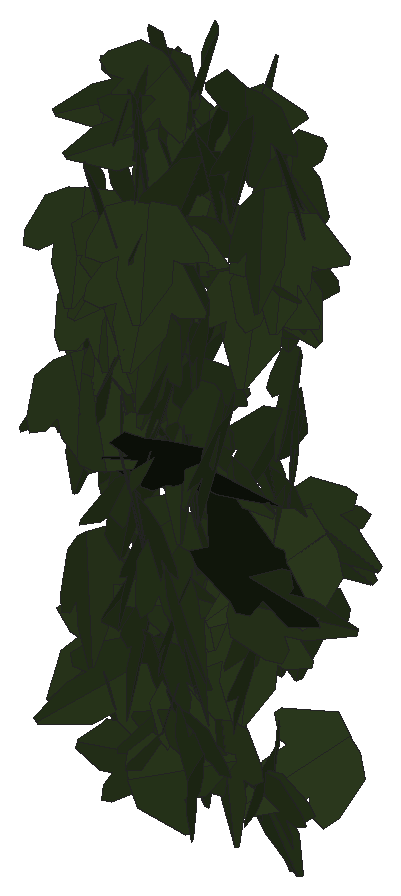
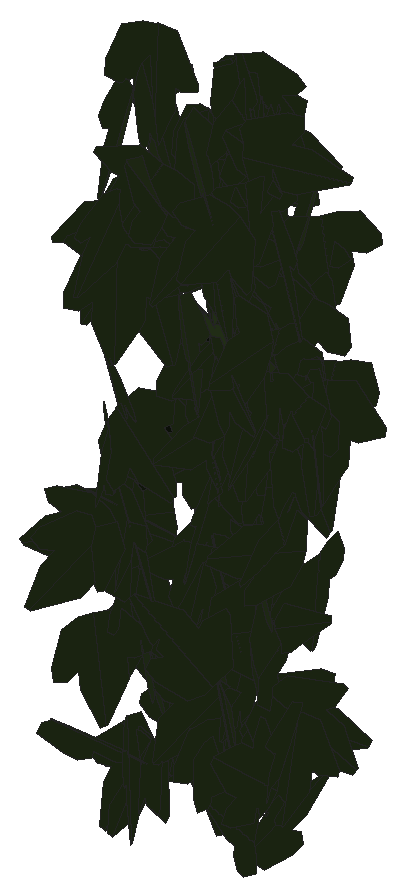
# SketchUp Ruby script. Lengths in inches.
U = 1.inch
M = Sketchup.active_model
def pt(a) = Geom::Point3d.new(a.map { |v| v * U })
def face(e, loops, mat)
  f = e.add_face(loops[0].map { |a| pt(a) })
  loops[1..].each { |l| e.add_face(l.map { |a| pt(a) }).erase! }
  f.material = f.back_material = mat if mat
  f
end
# faces: each face lists its corners as indices into pts; further lists are holes
def faces(e, pts, list, mat = nil) = list.each { |f| face(e, (f[0].is_a?(Array) ? f : [f]).map { |l| l.map { |i| pts[i] } }, mat) }
# xy, xz, yz: faces in a plane at the given z, y or x. An outline is a flat list of corners, or four numbers for a rectangle; further outlines are holes
def ring(l) = l.size == 4 ? [[l[0], l[1]], [l[2], l[1]], [l[2], l[3]], [l[0], l[3]]] : l.each_slice(2).to_a
def flat(e, list, mat, &to3) = list.each { |f| face(e, (f[0].is_a?(Array) ? f : [f]).map { |l| ring(l).map { |u, v| to3.(u, v) } }, mat) }
def xy(e, z, list, mat = nil) = flat(e, list, mat) { |x, y| [x, y, z] }
def xz(e, y, list, mat = nil) = flat(e, list, mat) { |x, z| [x, y, z] }
def yz(e, x, list, mat = nil) = flat(e, list, mat) { |y, z| [x, y, z] }
def lines(e, pts, list) = list.each { |a, b| e.add_line(pt(pts[a]), pt(pts[b])) }
# prism: a flat outline (further loops are holes) pulled along v
def prism(e, loops, v, mat = nil)
  f = face(e, loops, mat); d = Geom::Vector3d.new(v.map { |x| x * U })
  f.pushpull(f.normal.samedirection?(d) ? d.length : -d.length)
end
def box(e, o, s, mat = nil) = prism(e, [[o, [o[0] + s[0], o[1], o[2]], [o[0] + s[0], o[1] + s[1], o[2]], [o[0], o[1] + s[1], o[2]]]], [0, 0, s[2]], mat)
def at(x, y, z, deg = 0) = Geom::Transformation.translation(pt([x, y, z])) * Geom::Transformation.rotation(ORIGIN, Z_AXIS, deg.degrees)
def axes(o, x, y, z) = Geom::Transformation.new([*x, 0, *y, 0, *z, 0, *pt(o).to_a, 1])
def part(name) = M.definitions.add(name)
# library, detail: a bought-in or finely detailed component or shape, given as its bounding box
def library(name, o, s) = part(name).tap { |d| box(d.entities, o, s) }
def detail(e, o, s) = box(e.add_group.entities, o, s)
def put(e, d, t, mat = nil) = e.add_instance(d, t).tap { |i| i.material = mat if mat }
def group(e, t, mat = nil) = e.add_group.tap { |g| g.transformation = t; g.material = mat if mat }.entities
root = M.entities
M.materials.add("efeu1").color = [18, 25, 13]
M.materials.add("efeu2").color = [43, 57, 29]
c1 = part("ivyleaf_10")
p = [[0,0.5,-0.03],[-0.0625,2.02,-0.43],[-0.19,2.01,-0.46],[-0.54,1.05,-0.29],[-0.52,0.625,-0.18],[-0.83,0.76,-0.28],
  [-1.16,0.64,-0.33],[-1.15,0.33,-0.24],[-0.77,-0.39,0.02],[-0.3,-0.51,0.16],[0.04,-0.48,0.23],[-0.02,2.01,-0.4375],
  [-0.06,2.01,-0.43],[0.04,-0.49,0.23],[0.67,-0.49,0.14],[1.38,0.36,-0.2],[1.375,0.51,-0.24],[0.81,0.65,-0.19],
  [0.62,0.59,-0.15],[0.6,1.09,-0.28],[0.5,1.23,-0.31]]
faces(c1.entities,p,[[0,1,2,3,4,5,6,7,8,9,10],[11,12,0,13,14,15,16,17,18,19,20]],"efeu2")
c2 = part("ivyleaf_9")
p = [[1.54,2.16,1.25],[1.36,2.04,1.19],[-0.21,0.99,0.68],[-0.71,1.11,0.82],[-0.85,0.86,0.67],[-0.8,0.17,0.21],
  [-0.9,-0.01,0.1],[-0.67,-0.16,-0.02],[-0.08,-0.08,-0.05],[-0.03,-0.6,-0.4],[0.65,-0.88,-0.66],[0.83,-0.6,-0.49],
  [1.29,-0.42,-0.43],[1.8125,-0.07,-0.26],[1.21,0.44,0.15]]
faces(c2.entities,p,[[0,1,2,3,4,5,6,7,8,9,10,11,12,13,14]],"efeu1")
put(root,c1,axes([601.08,137.34,181.58],[0.64359,0.26762,0.03048],[0.02819,0.0116,-0.69701],[-0.26787,0.6442,-0.00012]))
put(root,c1,axes([600.44,137.24,177.87],[0.63198,0.08245,0.22157],[-0.22103,-0.01835,0.63726],[0.08389,-0.66944,0.00982]))
put(root,c1,axes([600.58,137.56,177.23],[0.21939,-0.51968,-0.31436],[0.29929,-0.19834,0.53676],[-0.5285,-0.32805,0.17347]))
put(root,c1,axes([602.34,137.49,178.65],[0.29087,-0.70755,-0.02213],[-0.00687,0.0211,-0.76501],[0.70787,0.29094,0.00166]))
put(root,c1,axes([600.9,137.21,177.67],[-0.44004,0.56978,0.24643],[-0.21023,0.14743,-0.71629],[-0.5841,-0.48231,0.07216]))
put(root,c1,axes([599.86,137.3,178.71],[0.39194,0.58267,0.14037],[0.01326,0.15926,-0.69806],[-0.59919,0.38466,0.07638]))
put(root,c1,axes([602.02,137.62,178.76],[0.57612,-0.4529,0.05393],[0.02997,-0.0491,-0.73255],[0.45511,0.57655,-0.02002]))
put(root,c1,axes([600.95,137.53,180.64],[0.65383,0.23933,-0.04503],[-0.04114,-0.01861,-0.69625],[-0.24002,0.65512,-0.00333]))
put(root,c1,axes([601.14,137.3,176.98],[-0.61616,0.38055,0.21329],[-0.19698,0.08664,-0.72364],[-0.38924,-0.64625,0.02858]))
put(root,c1,axes([599.96,137.52,175.73],[-0.01317,0.74417,-0.12889],[-0.02723,-0.12929,-0.74372],[-0.75476,-0.00832,0.02908]))
put(root,c1,axes([599.76,137.5625,181.25],[0.50641,0.45036,-0.05576],[-0.04149,-0.03726,-0.6777],[-0.4519,0.50811,-0.00027]))
put(root,c1,axes([601.09,137.65,179.69],[0.63288,-0.28069,0.04328],[0.03884,-0.01918,-0.69233],[0.28133,0.63407,-0.00178]))
put(root,c1,axes([600.625,137.1,179],[0.25813,-0.02662,0.66088],[-0.40034,0.55843,0.17886],[-0.5265,-0.43767,0.18801]))
put(root,c2,axes([601.01,137.22,177.88],[0.68224,0.09053,0.33278],[0.31417,0.14109,-0.68248],[-0.14224,0.74584,0.08871]))
put(root,c1,axes([600.31,137.66,180.9],[0.61475,0.08364,-0.24112],[-0.23926,-0.03001,-0.62041],[-0.08883,0.65966,0.00235]))
put(root,c1,axes([601.65,137.4,175.92],[-0.31683,0.67633,0.09582],[-0.02648,0.09339,-0.7467],[-0.68258,-0.31755,-0.01551]))
put(root,c1,axes([602.05,137.09,173.21],[0.20562,-0.1414,-0.71854],[-0.18335,0.71262,-0.1927],[0.709,0.2253,0.15855]))
put(root,c1,axes([600.09,137.49,181.77],[-0.49451,0.54874,-0.01723],[0.01053,-0.0137,-0.73869],[-0.54891,-0.49462,0.00135]))
put(root,c1,axes([600.61,137.67,177.11],[-0.06245,-0.6591,-0.00693],[0.0011,0.00686,-0.66205],[0.65914,-0.06246,0.00045]))
put(root,c1,axes([600.02,137.59,179.92],[0.56226,0.18794,0.34559],[0.3275,0.11033,-0.59284],[-0.21793,0.65069,0.00071]))
put(root,c1,axes([601.1875,137.82,179.01],[0.21612,-0.6216,0.13768],[0.04814,-0.12903,-0.65809],[0.63484,0.22139,0.00303]))
put(root,c1,axes([601.65,137.55,175.17],[-0.39505,0.62803,0.05802],[-0.03606,0.04586,-0.74193],[-0.62968,-0.39665,0.00609]))
put(root,c1,axes([599.64,137.64,178.49],[-0.18698,-0.67729,-0.21292],[0.04196,0.20925,-0.70248],[0.70873,-0.19107,-0.01459]))
put(root,c1,axes([600.45,138.11,174.61],[0.2108,-0.47067,0.42743],[0.29014,-0.32947,-0.5059],[0.56573,0.34436,0.10019]))
put(root,c1,axes([601.33,137.84,175.54],[0.37359,-0.63232,-0.08899],[-0.04891,0.07446,-0.73443],[0.63667,0.37676,-0.0042]))
put(root,c1,axes([600.7,137.96,182.74],[0.27723,0.10228,-0.58345],[-0.56766,-0.13819,-0.29395],[-0.16925,0.63101,0.0302]))
put(root,c1,axes([600.34,137.6875,178.41],[-0.38327,0.54407,0.22852],[-0.34026,0.01888,-0.61563],[-0.48214,-0.44582,0.25281]))
put(root,c1,axes([600.12,138.14,173.68],[0.23984,0.24368,-0.61379],[-0.50676,-0.3508,-0.33729],[-0.42344,0.55785,0.05601]))
put(root,c1,axes([601.13,138.03,177.81],[0.56401,-0.2282,0.32278],[0.30012,-0.11881,-0.60842],[0.25727,0.63888,0.00215]))
put(root,c2,axes([603,137.57,176.22],[-0.12417,0.8107,0.01601],[-0.80422,-0.1252,0.10223],[0.10347,-0.00022,0.81375]))
put(root,c1,axes([600.41,137.95,182.9375],[-0.38264,0.47354,-0.26209],[0.12867,-0.23218,-0.60736],[-0.52572,-0.40149,0.0421]))
put(root,c1,axes([599.71,138.15,178],[-0.04918,-0.68772,0.24142],[0.063,-0.24508,-0.68529],[0.72614,-0.02532,0.07581]))
put(root,c1,axes([600.81,138.34,181.45],[-0.06377,0.18585,-0.61505],[-0.04136,-0.61798,-0.18245],[-0.64119,0.02138,0.07294]))
put(root,c1,axes([600.83,137.83,172.4375],[0.25774,-0.08436,-0.62466],[0.6296,0.00193,0.25952],[-0.03038,-0.67575,0.07873]))
put(root,c1,axes([601.23,137.69,176.23],[0.10155,0.7108,0.20738],[-0.07922,0.21855,-0.71029],[-0.73618,0.07453,0.10504]))
put(root,c1,axes([600.75,138.02,183.59],[0.55972,-0.02827,-0.35294],[-0.35254,0.0169,-0.56044],[0.03293,0.66149,-0.00077]))
put(root,c1,axes([600.5,138.16,182.89],[-0.11887,0.51849,-0.36064],[0.03216,-0.36152,-0.53037],[-0.63076,-0.11615,0.04092]))
put(root,c1,axes([601.72,137.77,180.27],[0.43917,-0.41036,-0.44287],[-0.22721,0.39505,-0.59137],[0.55938,0.48264,0.10749]))
put(root,c1,axes([600.34,137.9375,178.5625],[-0.68695,-0.16614,0.01577],[-0.01539,-0.00342,-0.70676],[0.16618,-0.68712,-0.0003]))
put(root,c1,axes([600.76,138.02,175.31],[-0.14366,-0.00275,0.62823],[0.62503,0.06437,0.14321],[-0.06336,0.64122,-0.01169]))
put(root,c1,axes([600.2,138.08,179.125],[0.27265,0.57164,-0.16029],[-0.05782,-0.14998,-0.63322],[-0.59087,0.27845,-0.012]))
put(root,c1,axes([601.35,138.03,173.01],[-0.62254,-0.07937,0.30773],[-0.29055,-0.13208,-0.62184],[0.12876,-0.68176,0.08465]))
put(root,c1,axes([600.3125,138.22,175.92],[0.32857,-0.56663,0.16094],[0.08957,-0.13409,-0.65493],[0.5822,0.34041,0.00993]))
put(root,c1,axes([601.07,138.36,177.5625],[0.15591,-0.22218,0.57986],[0.49512,-0.31636,-0.25434],[0.37479,0.51036,0.09478]))
put(root,c1,axes([599.78,137.75,178.59],[0.34855,-0.36414,-0.55987],[-0.25985,0.50783,-0.49206],[0.61525,0.42077,0.10935]))
put(root,c1,axes([601.23,138.24,182.11],[-0.0277,-0.64316,0.16385],[-0.01515,-0.16334,-0.64371],[0.66353,-0.03058,-0.00785]))
put(root,c1,axes([601.14,138.11,180.21],[0.49807,-0.41094,-0.15334],[-0.11936,0.09628,-0.64571],[0.42207,0.51217,-0.00165]))
put(root,c1,axes([602.72,137.78,175.77],[0.18244,-0.09676,0.68328],[0.49793,0.5078,-0.06104],[-0.47782,0.49224,0.19728]))
put(root,c1,axes([600.84,138.03,174.33],[-0.65749,0.07766,-0.02077],[0.02274,0.01556,-0.66181],[-0.07711,-0.65763,-0.01811]))
put(root,c1,axes([599.77,138.43,173.96],[-0.38351,-0.23761,0.5026],[-0.30224,-0.42336,-0.43077],[0.4666,-0.46952,0.13407]))
put(root,c1,axes([600.28,138.06,179.46],[0.14218,0.62258,0.06943],[0.01644,0.06746,-0.6386],[-0.62622,0.14312,-0.001]))
put(root,c1,axes([601.3125,138.04,173.3],[-0.65995,0.25682,0.07306],[-0.06516,0.03401,-0.70812],[-0.25894,-0.66311,-0.00802]))
put(root,c1,axes([601.8,138.35,173.01],[-0.57561,0.26008,-0.27985],[0.1379,-0.3305,-0.5908],[-0.35628,-0.5481,0.22345]))
put(root,c1,axes([602.18,138.37,183.05],[0.16056,-0.68096,0.10617],[0.05677,-0.09557,-0.69886],[0.68684,0.16708,0.03295]))
put(root,c1,axes([600.33,138.375,175.86],[0.00874,0.00964,-0.64829],[0.57065,-0.30789,0.00312],[-0.30779,-0.57057,-0.01263]))
put(root,c1,axes([600.64,138.09,181.14],[-0.25887,-0.29696,-0.51076],[0.53223,0.12488,-0.34236],[0.2565,-0.55883,0.1949]))
put(root,c1,axes([599.89,138.75,174.8125],[-0.03806,-0.05106,-0.69109],[0.04477,-0.69087,0.04858],[-0.69153,-0.04191,0.04118]))
put(root,c1,axes([601.16,138.07,177.37],[-0.21351,0.27092,-0.57718],[-0.52137,0.27619,0.3225],[0.36702,0.54995,0.12237]))
put(root,c1,axes([600.91,138.39,172.78],[-0.08931,-0.63325,0.0927],[-0.02657,-0.08985,-0.63937],[0.63945,-0.09218,-0.01362]))
put(root,c1,axes([600.13,138.09,181.25],[0.35851,-0.44174,-0.4577],[-0.2748,0.36628,-0.56875],[0.57368,0.4515,0.01359]))
put(root,c1,axes([599.62,138.25,178.78],[0.52407,0.15019,0.40597],[0.38306,0.13593,-0.54479],[-0.20157,0.64883,0.02016]))
put(root,c1,axes([602.26,138.26,183.57],[-0.70324,0.07976,0.12362],[-0.12968,-0.05094,-0.70482],[-0.06949,-0.7122,0.06426]))
put(root,c1,axes([602.87,138.71,176.32],[-0.68465,0.30675,0.33162],[-0.42647,-0.63747,-0.29081],[0.14897,-0.41515,0.69157]))
put(root,c1,axes([600.77,138.11,182.6],[-0.06574,0.01768,0.64973],[-0.6265,0.1722,-0.06808],[-0.1731,-0.62994,-0.00037]))
put(root,c1,axes([600.55,138.56,175.02],[-0.09266,-0.03208,-0.65813],[-0.62184,-0.21552,0.09806],[-0.21789,0.62871,0.00003]))
put(root,c1,axes([601.22,138.29,178.89],[-0.63732,-0.16943,0.08223],[-0.07893,-0.02317,-0.65945],[0.17099,-0.64219,0.0021]))
put(root,c1,axes([600.94,138.34,172.99],[-0.3896,-0.51808,-0.01696],[0.01934,0.00667,-0.64812],[0.518,-0.38991,0.01145]))
put(root,c1,axes([600.52,138.55,183.35],[0.02575,0.53188,-0.34971],[-0.12355,-0.33917,-0.52493],[-0.62444,0.08904,0.08944]))
put(root,c1,axes([599.82,138.73,172.01],[-0.13969,0.33649,0.52486],[0.05595,-0.52893,0.354],[0.62094,0.12336,0.08617]))
put(root,c1,axes([600.48,138.34,178.49],[-0.60779,-0.23896,0.03297],[-0.02904,-0.01623,-0.65306],[0.23947,-0.60847,0.00447]))
put(root,c1,axes([600.95,138.43,181.01],[-0.48309,-0.39821,0.12112],[-0.09552,-0.07454,-0.62605],[0.40512,-0.49243,-0.00318]))
put(root,c1,axes([600.79,138.28,183.62],[-0.50459,0.26111,0.3322],[-0.3499,0.03184,-0.55651],[-0.23686,-0.60329,0.11441]))
put(root,c1,axes([601.4375,138.26,182.55],[-0.54868,0.35966,0.15997],[-0.13624,0.08396,-0.65604],[-0.3693,-0.56532,0.00434]))
put(root,c1,axes([601.17,138.36,175.8],[0.48033,0.4413,0.14869],[0.10109,0.1097,-0.65217],[-0.45457,0.49071,0.01208]))
put(root,c1,axes([600.1,138.71,182.82],[0.19129,0.08868,-0.65033],[-0.59725,-0.2574,-0.21077],[-0.27219,0.62711,0.00545]))
put(root,c1,axes([601.29,138.24,176.88],[-0.35904,0.52398,0.21858],[-0.12367,0.18023,-0.63519],[-0.5541,-0.37974,0.00013]))
put(root,c1,axes([601.29,138.43,177.4375],[0.21496,-0.05663,0.60563],[0.59493,0.15335,-0.19683],[-0.12668,0.62408,0.10332]))
put(root,c1,axes([599.66,138.41,173.6],[-0.65579,-0.02069,0.03525],[-0.03497,-0.00937,-0.65606],[0.02116,-0.65667,0.00825]))
put(root,c1,axes([600.1875,138.23,182.42],[0.11513,-0.47739,0.43153],[-0.11393,0.41633,0.49098],[-0.63336,-0.16167,-0.00988]))
put(root,c1,axes([600.39,138.89,179.41],[-0.02877,-0.22617,-0.60564],[0.35501,-0.51218,0.17441],[-0.5403,-0.32449,0.14684]))
put(root,c1,axes([601.97,138.67,174.39],[0.29664,-0.61041,0.08633],[0.06745,-0.06309,-0.67787],[0.61278,0.30243,0.03283]))
put(root,c1,axes([602.1,138.57,180.33],[0.59016,0.3555,-0.04267],[-0.03955,-0.01704,-0.68894],[-0.35586,0.59145,0.0058]))
put(root,c1,axes([601.23,138.55,182.63],[0.04032,-0.63697,-0.09723],[-0.01188,0.09667,-0.63822],[0.64424,0.04165,-0.00569]))
put(root,c1,axes([599.64,138.74,177.04],[0.00995,0.56322,-0.30632],[0.00243,-0.30639,-0.56327],[-0.64113,0.00758,-0.00689]))
put(root,c1,axes([602.25,138.6,181.63],[0.08586,0.68528,-0.11861],[-0.08817,-0.10782,-0.68676],[-0.68986,0.09907,0.07301]))
put(root,c1,axes([601.17,138.07,179.11],[0.08041,-0.04179,-0.68303],[0.03064,0.68726,-0.03844],[0.68362,-0.02589,0.08207]))
put(root,c1,axes([601.08,138.35,173.63],[0.33259,0.39263,0.41411],[0.2601,0.32233,-0.51451],[-0.50793,0.42215,0.00769]))
put(root,c1,axes([602.25,138.57,172.37],[-0.61697,0.11882,-0.22736],[0.21482,-0.08443,-0.62704],[-0.14023,-0.65208,0.03976]))
put(root,c1,axes([600.72,138.54,173.76],[0.33052,-0.5172,-0.22841],[-0.10751,0.20225,-0.61355],[0.55507,0.34715,0.01717]))
put(root,c1,axes([602.13,138.65,180.26],[-0.58104,-0.23408,0.27559],[-0.24762,-0.12253,-0.62612],[0.2635,-0.6313,0.01933]))
put(root,c1,axes([600.29,138.14,178.51],[-0.12944,0.28389,0.59825],[-0.2626,0.53759,-0.31192],[-0.6079,-0.29267,0.00736]))
put(root,c1,axes([601.91,138.67,174.73],[0.62379,0.28945,0.00194],[0.00693,-0.01033,-0.68757],[-0.28938,0.62371,-0.01229]))
put(root,c1,axes([602.25,138.57,172.42],[-0.60712,0.26115,-0.10228],[0.09481,-0.03841,-0.6609],[-0.26395,-0.61448,-0.00215]))
put(root,c1,axes([599.67,138.39,173.75],[-0.23602,0.50899,0.31432],[-0.16153,0.27113,-0.56034],[-0.57601,-0.28459,0.02834]))
put(root,c1,axes([601.32,138.58,174.72],[0.06926,0.64521,-0.07355],[-0.02451,0.07651,0.64811],[0.64892,-0.06597,0.03233]))
put(root,c1,axes([600.17,138.76,182.18],[0.36118,0.5389,-0.07464],[-0.038,-0.06438,-0.64873],[-0.54272,0.36315,-0.00424]))
put(root,c1,axes([602.05,139.02,177.94],[-0.09576,-0.59082,0.30295],[-0.04356,-0.29983,-0.59851],[0.66253,-0.1051,0.00444]))
put(root,c1,axes([600.99,138.28,178.07],[-0.03959,-0.08426,-0.63753],[0.22102,0.59804,-0.09277],[0.6039,-0.2244,-0.00785]))
put(root,c1,axes([600.92,138.49,180.77],[0.35546,-0.15738,-0.51242],[-0.29459,0.45631,-0.3445],[0.44783,0.42509,0.1801]))
put(root,c1,axes([602.51,138.64,182.7],[-0.48902,0.49137,0.06251],[-0.03792,0.05045,-0.69319],[-0.49387,-0.49041,-0.00867]))
put(root,c1,axes([601.27,138.73,179.82],[0.2373,-0.54857,-0.22597],[-0.09446,0.20534,-0.59767],[0.58572,0.25536,-0.00484]))
put(root,c1,axes([602.23,138.75,172.73],[0.22606,-0.61594,-0.22684],[-0.00985,0.23671,-0.65255],[0.65631,0.21571,0.06834]))
put(root,c1,axes([602.12,138.73,175.15],[0.01622,-0.64952,-0.24261],[0.10847,0.24206,-0.64081],[0.68481,-0.02296,0.10725]))
put(root,c1,axes([602.375,138.88,181.19],[0.43389,0.52433,-0.07138],[-0.0483,-0.05268,-0.68056],[-0.52695,0.43655,0.00361]))
put(root,c1,axes([602.87,139.26,172.83],[-0.62233,0.29011,0.36104],[-0.42272,-0.6029,-0.24419],[0.18927,-0.39263,0.64174]))
put(root,c1,axes([602.3,139.12,178.91],[0.48532,-0.39807,0.16573],[0.13415,-0.09775,-0.62762],[0.40979,0.50343,0.00918]))
put(root,c1,axes([600.98,138.58,181.29],[0.11233,0.42379,0.47531],[0.03717,0.47747,-0.43449],[-0.63572,0.1028,0.05858]))
put(root,c1,axes([602.23,138.71,180.69],[0.27176,0.53,0.36014],[0.12752,0.33864,-0.59458],[-0.62797,0.29813,0.03512]))
put(root,c1,axes([599.71,138.54,176.5625],[0.05868,-0.20788,0.63337],[0.00927,0.63601,0.20788],[-0.66655,-0.00945,0.05865]))
put(root,c1,axes([599.76,139.26,172.34],[0.01465,-0.07944,0.63931],[0.62769,-0.14218,-0.03205],[0.14501,0.62347,0.07415]))
put(root,c1,axes([602.26,139.07,180.4],[-0.43993,-0.49602,-0.01808],[0.01189,0.01362,-0.663],[0.49621,-0.44009,-0.00015]))
put(root,c1,axes([601.91,139.22,176.83],[0.43366,-0.42287,-0.2621],[-0.17298,0.19784,-0.6054],[0.46647,0.46649,0.01916]))
put(root,c1,axes([601.96,139.25,176.88],[-0.59553,0.28618,0.04859],[-0.06405,-0.02137,-0.65906],[-0.28313,-0.59713,0.04688]))
put(root,c1,axes([600.61,139.3,174.74],[-0.40177,-0.16736,0.49239],[0.45391,0.19083,0.43523],[-0.25382,0.60617,-0.00107]))
put(root,c1,axes([602.07,139.55,177.95],[-0.31547,0.49004,-0.26927],[0.00285,-0.30776,-0.56342],[-0.55914,-0.27805,0.14905]))
put(root,c1,axes([600.49,139.52,183.25],[0.317,-0.55651,0.01484],[0.01141,-0.01058,-0.64044],[0.55659,0.31717,0.00468]))
put(root,c1,axes([599.63,139.15,173.14],[0.1064,-0.42627,0.46938],[-0.12224,0.45322,0.43931],[-0.62216,-0.16195,-0.00604]))
put(root,c1,axes([602.3,139.5,176.47],[-0.31394,-0.01895,-0.5643],[0.56162,-0.07697,-0.30986],[-0.05815,-0.64115,0.05388]))
put(root,c1,axes([599.94,139.55,182.0625],[-0.53503,0.05999,-0.33972],[0.32728,-0.10993,-0.53485],[-0.10907,-0.62416,0.06155]))
put(root,c1,axes([599.75,139.09,180.01],[0.09139,-0.06144,0.63775],[-0.23889,0.59448,0.0915],[-0.5945,-0.24833,0.06127]))
put(root,c1,axes([602.18,139.62,174.81],[-0.31195,-0.55563,0.04178],[-0.01276,-0.04075,-0.63715],[0.55705,-0.31208,0.00881]))
put(root,c1,axes([601.2,139.52,182.48],[0.51327,0.2033,0.33282],[0.29516,0.15706,-0.55114],[-0.2549,0.59123,0.03197]))
put(root,c1,axes([602.32,139.52,176.21],[-0.42427,-0.26028,-0.40786],[0.36182,0.18947,-0.49728],[0.32123,-0.55719,0.02142]))
put(root,c1,axes([601.22,139.52,182.01],[0.2579,-0.47607,0.34173],[-0.17245,0.29518,0.54136],[-0.56007,-0.3101,-0.00932]))
put(root,c1,axes([600.0625,139.52,179.72],[-0.06716,0.1069,0.6259],[-0.60497,0.18038,-0.09572],[-0.19284,-0.60309,0.08231]))
put(root,c1,axes([601.74,139.6875,181.77],[-0.09891,-0.54731,-0.31172],[0.22731,0.26326,-0.53435],[0.58741,-0.19403,0.15429]))
